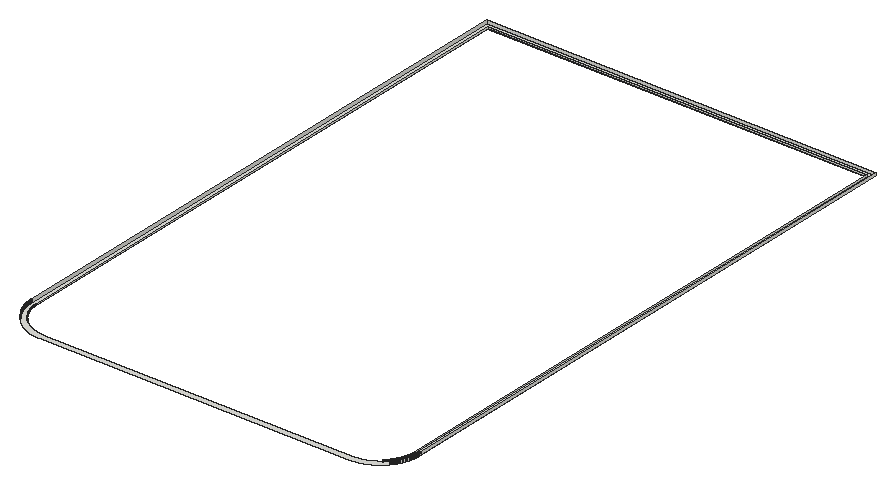
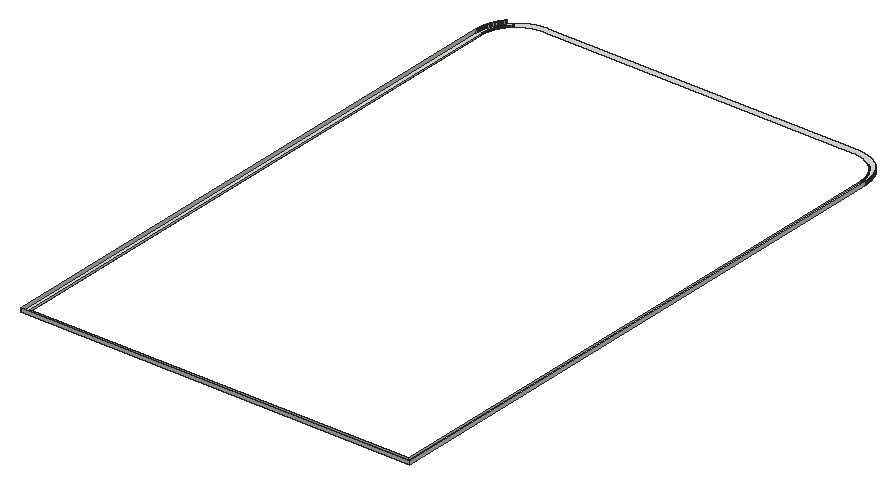
# SketchUp Ruby script. Lengths in inches.
U = 1.inch
M = Sketchup.active_model
def pt(a) = Geom::Point3d.new(a.map { |v| v * U })
def face(e, loops, mat)
  f = e.add_face(loops[0].map { |a| pt(a) })
  loops[1..].each { |l| e.add_face(l.map { |a| pt(a) }).erase! }
  f.material = f.back_material = mat if mat
  f
end
# faces: each face lists its corners as indices into pts; further lists are holes
def faces(e, pts, list, mat = nil) = list.each { |f| face(e, (f[0].is_a?(Array) ? f : [f]).map { |l| l.map { |i| pts[i] } }, mat) }
# xy, xz, yz: faces in a plane at the given z, y or x. An outline is a flat list of corners, or four numbers for a rectangle; further outlines are holes
def ring(l) = l.size == 4 ? [[l[0], l[1]], [l[2], l[1]], [l[2], l[3]], [l[0], l[3]]] : l.each_slice(2).to_a
def flat(e, list, mat, &to3) = list.each { |f| face(e, (f[0].is_a?(Array) ? f : [f]).map { |l| ring(l).map { |u, v| to3.(u, v) } }, mat) }
def xy(e, z, list, mat = nil) = flat(e, list, mat) { |x, y| [x, y, z] }
def xz(e, y, list, mat = nil) = flat(e, list, mat) { |x, z| [x, y, z] }
def yz(e, x, list, mat = nil) = flat(e, list, mat) { |y, z| [x, y, z] }
def lines(e, pts, list) = list.each { |a, b| e.add_line(pt(pts[a]), pt(pts[b])) }
# prism: a flat outline (further loops are holes) pulled along v
def prism(e, loops, v, mat = nil)
  f = face(e, loops, mat); d = Geom::Vector3d.new(v.map { |x| x * U })
  f.pushpull(f.normal.samedirection?(d) ? d.length : -d.length)
end
def box(e, o, s, mat = nil) = prism(e, [[o, [o[0] + s[0], o[1], o[2]], [o[0] + s[0], o[1] + s[1], o[2]], [o[0], o[1] + s[1], o[2]]]], [0, 0, s[2]], mat)
def at(x, y, z, deg = 0) = Geom::Transformation.translation(pt([x, y, z])) * Geom::Transformation.rotation(ORIGIN, Z_AXIS, deg.degrees)
def axes(o, x, y, z) = Geom::Transformation.new([*x, 0, *y, 0, *z, 0, *pt(o).to_a, 1])
def part(name) = M.definitions.add(name)
# library, detail: a bought-in or finely detailed component or shape, given as its bounding box
def library(name, o, s) = part(name).tap { |d| box(d.entities, o, s) }
def detail(e, o, s) = box(e.add_group.entities, o, s)
def put(e, d, t, mat = nil) = e.add_instance(d, t).tap { |i| i.material = mat if mat }
def group(e, t, mat = nil) = e.add_group.tap { |g| g.transformation = t; g.material = mat if mat }.entities
root = M.entities
xy(root,347,[[[38.61,204,38.21,204.01,37.82,204.02,37.43,204.04,37.04,204.0625,36.65,204.09,36.25,204.125,35.86,204.16,35.08,204.26,34.7,204.31,33.92,204.43,33.53,204.5,33.15,204.58,32.76,204.66,32.38,204.74,31.62,204.92,31.24,205.02,30.86,205.125,30.48,205.24,30.1,205.35,29.36,205.59,28.62,205.85,28.25,205.99,27.88,206.14,27.52,206.28,27.16,206.4375,26.8,206.59,26.44,206.76,26.08,206.92,25.73,207.09,25.03,207.45,24.69,207.64,24.34,207.83,24,208.02,23.66,208.22,23.33,208.42,22.99,208.63,22.66,208.84,22.33,209.06,22.01,209.28,21.6875,209.5,21.37,209.73,21.05,209.96,20.43,210.44,20.12,210.6875,19.82,210.93,19.52,211.1875,19.22,211.44,18.93,211.71,18.64,211.97,18.35,212.24,18.07,212.51,17.51,213.07,17.24,213.35,16.97,213.64,16.71,213.93,16.44,214.22,16.1875,214.52,15.93,214.82,15.6875,215.12,15.44,215.43,14.96,216.05,14.73,216.37,14.5,216.6875,14.28,217.01,14.06,217.33,13.84,217.66,13.63,217.99,13.42,218.33,13.22,218.66,13.02,219,12.83,219.34,12.64,219.69,12.45,220.03,12.09,220.73,11.92,221.08,11.76,221.44,11.59,221.8,11.4375,222.16,11.28,222.52,11.14,222.88,10.99,223.25,10.85,223.62,10.59,224.36,10.35,225.1,10.24,225.48,10.125,225.86,10.02,226.24,9.92,226.62,9.74,227.38,9.66,227.76,9.58,228.15,9.5,228.53,9.43,228.92,9.31,229.7,9.26,230.08,9.16,230.86,9.125,231.25,9.09,231.65,9.0625,232.04,9.04,232.43,9.02,232.82,9.01,233.21,9,233.61,9,660,300,660,300,233.61,299.99,233.21,299.98,232.82,299.96,232.43,299.9375,232.04,299.91,231.65,299.875,231.25,299.84,230.86,299.74,230.08,299.69,229.7,299.57,228.92,299.5,228.53,299.42,228.15,299.34,227.76,299.26,227.38,299.08,226.62,298.98,226.24,298.875,225.86,298.76,225.48,298.65,225.1,298.41,224.36,298.15,223.62,298.01,223.25,297.86,222.88,297.72,222.52,297.5625,222.16,297.41,221.8,297.24,221.44,297.08,221.08,296.91,220.73,296.55,220.03,296.36,219.69,296.17,219.34,295.98,219,295.78,218.66,295.58,218.33,295.37,217.99,295.16,217.66,294.94,217.33,294.72,217.01,294.5,216.6875,294.27,216.37,294.04,216.05,293.56,215.43,293.3125,215.12,293.07,214.82,292.8125,214.52,292.56,214.22,292.29,213.93,292.03,213.64,291.76,213.35,291.49,213.07,290.93,212.51,290.65,212.24,290.36,211.97,290.07,211.71,289.78,211.44,289.48,211.1875,289.18,210.93,288.88,210.6875,288.57,210.44,287.95,209.96,287.63,209.73,287.3125,209.5,286.99,209.28,286.67,209.06,286.34,208.84,286.01,208.63,285.67,208.42,285.34,208.22,285,208.02,284.66,207.83,284.31,207.64,283.97,207.45,283.27,207.09,282.92,206.92,282.56,206.76,282.2,206.59,281.84,206.4375,281.48,206.28,281.12,206.14,280.75,205.99,280.38,205.85,279.64,205.59,278.9,205.35,278.52,205.24,278.14,205.125,277.76,205.02,277.38,204.92,276.62,204.74,276.24,204.66,275.85,204.58,275.47,204.5,275.08,204.43,274.3,204.31,273.92,204.26,273.14,204.16,272.75,204.125,272.35,204.09,271.96,204.0625,271.57,204.04,271.18,204.02,270.79,204.01,270.39,204],[38.66,208,270.34,208,271.02,208.02,272.04,208.08,272.72,208.14,273.06,208.18,273.39,208.22,274.07,208.32,274.4,208.375,274.74,208.44,275.07,208.5,275.41,208.57,275.74,208.64,276.4,208.8,277.06,208.98,277.38,209.07,277.71,209.17,278.03,209.27,278.36,209.38,278.68,209.49,279.32,209.73,279.63,209.85,279.95,209.98,280.26,210.11,280.58,210.25,280.89,210.39,281.19,210.53,281.5,210.68,281.8,210.83,282.11,210.99,282.41,211.15,282.7,211.32,283,211.48,283.29,211.66,283.58,211.83,283.875,212.01,284.16,212.19,284.44,212.38,284.73,212.57,285.01,212.77,285.28,212.97,285.56,213.17,285.83,213.37,286.1,213.58,286.36,213.79,286.89,214.23,287.14,214.45,287.4,214.68,287.9,215.14,288.14,215.375,288.38,215.62,288.625,215.86,288.86,216.1,289.32,216.6,289.55,216.86,289.77,217.11,290.21,217.64,290.42,217.9,290.63,218.17,290.83,218.44,291.03,218.72,291.23,218.99,291.43,219.27,291.62,219.56,291.81,219.84,291.99,220.125,292.17,220.42,292.34,220.71,292.52,221,292.68,221.3,292.85,221.59,293.01,221.89,293.17,222.2,293.32,222.5,293.47,222.81,293.61,223.11,293.75,223.42,293.89,223.74,294.02,224.05,294.15,224.37,294.27,224.68,294.51,225.32,294.62,225.64,294.73,225.97,294.83,226.29,294.93,226.62,295.02,226.94,295.2,227.6,295.36,228.26,295.43,228.59,295.5,228.93,295.56,229.26,295.625,229.6,295.68,229.93,295.78,230.61,295.82,230.94,295.86,231.28,295.92,231.96,295.98,232.98,296,233.66,296,656,13,656,13,233.66,13.02,232.98,13.08,231.96,13.14,231.28,13.18,230.94,13.22,230.61,13.32,229.93,13.375,229.6,13.44,229.26,13.5,228.93,13.57,228.59,13.64,228.26,13.8,227.6,13.98,226.94,14.07,226.62,14.17,226.29,14.27,225.97,14.38,225.64,14.49,225.32,14.73,224.68,14.85,224.37,14.98,224.05,15.11,223.74,15.25,223.42,15.39,223.11,15.53,222.81,15.68,222.5,15.83,222.2,15.99,221.89,16.15,221.59,16.32,221.3,16.48,221,16.66,220.71,16.83,220.42,17.01,220.125,17.19,219.84,17.38,219.56,17.57,219.27,17.77,218.99,17.97,218.72,18.17,218.44,18.37,218.17,18.58,217.9,18.79,217.64,19.23,217.11,19.45,216.86,19.68,216.6,20.14,216.1,20.375,215.86,20.62,215.62,20.86,215.375,21.1,215.14,21.6,214.68,21.86,214.45,22.11,214.23,22.64,213.79,22.9,213.58,23.17,213.37,23.44,213.17,23.72,212.97,23.99,212.77,24.27,212.57,24.56,212.38,24.84,212.19,25.125,212.01,25.42,211.83,25.71,211.66,26,211.48,26.3,211.32,26.59,211.15,26.89,210.99,27.2,210.83,27.5,210.68,27.81,210.53,28.11,210.39,28.42,210.25,28.74,210.11,29.05,209.98,29.37,209.85,29.68,209.73,30.32,209.49,30.64,209.38,30.97,209.27,31.29,209.17,31.62,209.07,31.94,208.98,32.6,208.8,33.26,208.64,33.59,208.57,33.93,208.5,34.26,208.44,34.6,208.375,34.93,208.32,35.61,208.22,35.94,208.18,36.28,208.14,36.96,208.08,37.98,208.02]]])
xz(root,656,[[13,347,296,348]])
xz(root,660,[[9,347,300,349.5]])
yz(root,9,[[233.61,347,234,349.5],[234,347,660,349.5]])
yz(root,13,[[233.66,347,234,348],[234,347,656,348]])
yz(root,296,[[233.66,347,234,348],[234,347,656,348]])
yz(root,300,[[233.61,347,234,349.5],[234,347,660,349.5]])
p = [[16.1875,214.52,349.5],[15.93,214.82,349.5],[15.93,214.82,347],[16.1875,214.52,347],[21.86,214.45,347],[21.6,214.68,347],
  [21.6,214.68,348],[21.86,214.45,348],[287.4,214.68,347],[287.14,214.45,347],[287.14,214.45,348],[287.4,214.68,348],
  [293.07,214.82,349.5],[292.8125,214.52,349.5],[292.8125,214.52,347],[293.07,214.82,347],[21.35,214.91,347],[21.35,214.91,348],
  [287.65,214.91,347],[287.65,214.91,348],[15.6875,215.12,349.5],[15.6875,215.12,347],[293.3125,215.12,349.5],[293.3125,215.12,347],
  [21.1,215.14,347],[21.1,215.14,348],[287.9,215.14,347],[287.9,215.14,348],[15.44,215.43,349.5],[15.44,215.43,347],
  [20.86,215.375,347],[20.86,215.375,348],[288.14,215.375,347],[288.14,215.375,348],[293.56,215.43,349.5],[293.56,215.43,347],
  [15.2,215.74,349.5],[15.2,215.74,347],[20.62,215.62,347],[20.62,215.62,348],[288.38,215.62,347],[288.38,215.62,348],
  [293.8,215.74,349.5],[293.8,215.74,347],[20.375,215.86,347],[20.375,215.86,348],[288.625,215.86,347],[288.625,215.86,348],
  [14.96,216.05,349.5],[14.96,216.05,347],[294.04,216.05,349.5],[294.04,216.05,347],[20.14,216.1,347],[20.14,216.1,348],
  [288.86,216.1,347],[288.86,216.1,348],[14.73,216.37,349.5],[14.73,216.37,347],[19.91,216.35,347],[19.91,216.35,348],
  [289.09,216.35,347],[289.09,216.35,348],[294.27,216.37,349.5],[294.27,216.37,347],[14.5,216.6875,349.5],[14.5,216.6875,347],
  [19.68,216.6,347],[19.68,216.6,348],[289.32,216.6,347],[289.32,216.6,348],[294.5,216.6875,349.5],[294.5,216.6875,347],
  [19.45,216.86,347],[19.45,216.86,348],[289.55,216.86,347],[289.55,216.86,348],[14.28,217.01,349.5],[14.28,217.01,347],
  [294.72,217.01,349.5],[294.72,217.01,347],[19.23,217.11,347],[19.23,217.11,348],[289.77,217.11,347],[289.77,217.11,348],
  [14.06,217.33,349.5],[14.06,217.33,347],[294.94,217.33,349.5],[294.94,217.33,347],[19.01,217.375,347],[19.01,217.375,348],
  [289.99,217.375,347],[289.99,217.375,348],[13.84,217.66,349.5],[13.84,217.66,347],[295.16,217.66,349.5],[295.16,217.66,347],
  [18.79,217.64,347],[18.79,217.64,348],[290.21,217.64,347],[290.21,217.64,348],[18.58,217.9,347],[18.58,217.9,348],
  [290.42,217.9,347],[290.42,217.9,348],[13.63,217.99,349.5],[13.63,217.99,347],[295.37,217.99,349.5],[295.37,217.99,347],
  [18.37,218.17,347],[18.37,218.17,348],[290.63,218.17,347],[290.63,218.17,348],[13.42,218.33,349.5],[13.42,218.33,347],
  [295.58,218.33,349.5],[295.58,218.33,347],[18.17,218.44,347],[18.17,218.44,348],[290.83,218.44,347],[290.83,218.44,348],
  [13.22,218.66,349.5],[13.22,218.66,347],[295.78,218.66,349.5],[295.78,218.66,347],[17.97,218.72,347],[17.97,218.72,348],
  [291.03,218.72,347],[291.03,218.72,348],[13.02,219,349.5],[13.02,219,347],[17.77,218.99,347],[17.77,218.99,348],
  [291.23,218.99,347],[291.23,218.99,348],[295.98,219,349.5],[295.98,219,347],[12.83,219.34,349.5],[12.83,219.34,347],
  [17.57,219.27,347],[17.57,219.27,348],[291.43,219.27,347],[291.43,219.27,348],[296.17,219.34,349.5],[296.17,219.34,347],
  [12.64,219.69,349.5],[12.64,219.69,347],[17.38,219.56,347],[17.38,219.56,348],[291.62,219.56,347],[291.62,219.56,348],
  [296.36,219.69,349.5],[296.36,219.69,347],[17.19,219.84,347],[17.19,219.84,348],[291.81,219.84,347],[291.81,219.84,348],
  [12.45,220.03,349.5],[12.45,220.03,347],[296.55,220.03,349.5],[296.55,220.03,347],[17.01,220.125,347],[17.01,220.125,348],
  [291.99,220.125,347],[291.99,220.125,348],[12.27,220.38,349.5],[12.27,220.38,347],[296.73,220.38,349.5],[296.73,220.38,347],
  [16.83,220.42,347],[16.83,220.42,348],[292.17,220.42,347],[292.17,220.42,348],[12.09,220.73,349.5],[12.09,220.73,347],
  [16.66,220.71,347],[16.66,220.71,348],[292.34,220.71,347],[292.34,220.71,348],[296.91,220.73,349.5],[296.91,220.73,347],
  [11.92,221.08,349.5],[11.92,221.08,347],[16.48,221,347],[16.48,221,348],[292.52,221,347],[292.52,221,348],
  [297.08,221.08,349.5],[297.08,221.08,347],[16.32,221.3,347],[16.32,221.3,348],[292.68,221.3,347],[292.68,221.3,348],
  [11.76,221.44,349.5],[11.76,221.44,347],[297.24,221.44,349.5],[297.24,221.44,347],[16.15,221.59,347],[16.15,221.59,348],
  [292.85,221.59,347],[292.85,221.59,348],[11.59,221.8,349.5],[11.59,221.8,347],[297.41,221.8,349.5],[297.41,221.8,347],
  [15.99,221.89,347],[15.99,221.89,348],[293.01,221.89,347],[293.01,221.89,348],[11.4375,222.16,349.5],[11.4375,222.16,347],
  [297.5625,222.16,349.5],[297.5625,222.16,347],[15.83,222.2,347],[15.83,222.2,348],[293.17,222.2,347],[293.17,222.2,348],
  [11.28,222.52,349.5],[11.28,222.52,347],[15.68,222.5,347],[15.68,222.5,348],[293.32,222.5,347],[293.32,222.5,348],
  [297.72,222.52,349.5],[297.72,222.52,347],[11.14,222.88,349.5],[11.14,222.88,347],[15.53,222.81,347],[15.53,222.81,348],
  [293.47,222.81,347],[293.47,222.81,348],[297.86,222.88,349.5],[297.86,222.88,347],[15.39,223.11,347],[15.39,223.11,348],
  [293.61,223.11,347],[293.61,223.11,348],[10.99,223.25,349.5],[10.99,223.25,347],[298.01,223.25,349.5],[298.01,223.25,347],
  [15.25,223.42,347],[15.25,223.42,348],[293.75,223.42,347],[293.75,223.42,348],[10.85,223.62,349.5],[10.85,223.62,347],
  [298.15,223.62,349.5],[298.15,223.62,347],[15.11,223.74,347],[15.11,223.74,348],[293.89,223.74,347],[293.89,223.74,348],
  [10.72,223.99,349.5],[10.72,223.99,347],[298.28,223.99,349.5],[298.28,223.99,347],[14.98,224.05,347],[14.98,224.05,348],
  [294.02,224.05,347],[294.02,224.05,348],[10.59,224.36,349.5],[10.59,224.36,347],[298.41,224.36,349.5],[298.41,224.36,347],
  [14.85,224.37,347],[14.85,224.37,348],[294.15,224.37,347],[294.15,224.37,348],[10.47,224.73,349.5],[10.47,224.73,347],
  [14.73,224.68,347],[14.73,224.68,348],[294.27,224.68,347],[294.27,224.68,348],[298.53,224.73,349.5],[298.53,224.73,347],
  [10.35,225.1,349.5],[10.35,225.1,347],[14.61,225,347],[14.61,225,348],[294.39,225,347],[294.39,225,348],
  [298.65,225.1,349.5],[298.65,225.1,347],[14.49,225.32,347],[14.49,225.32,348],[294.51,225.32,347],[294.51,225.32,348],
  [10.24,225.48,349.5],[10.24,225.48,347],[298.76,225.48,349.5],[298.76,225.48,347],[14.38,225.64,347],[14.38,225.64,348],
  [294.62,225.64,347],[294.62,225.64,348],[10.125,225.86,349.5],[10.125,225.86,347],[298.875,225.86,349.5],[298.875,225.86,347],
  [14.27,225.97,347],[14.27,225.97,348],[294.73,225.97,347],[294.73,225.97,348],[10.02,226.24,349.5],[10.02,226.24,347],
  [298.98,226.24,349.5],[298.98,226.24,347],[14.17,226.29,347],[14.17,226.29,348],[294.83,226.29,347],[294.83,226.29,348],
  [9.92,226.62,349.5],[9.92,226.62,347],[299.08,226.62,349.5],[299.08,226.62,347],[14.07,226.62,347],[14.07,226.62,348],
  [294.93,226.62,347],[294.93,226.62,348],[9.83,227,349.5],[9.83,227,347],[13.98,226.94,347],[13.98,226.94,348],
  [295.02,226.94,347],[295.02,226.94,348],[299.17,227,349.5],[299.17,227,347],[13.89,227.27,347],[13.89,227.27,348],
  [295.11,227.27,347],[295.11,227.27,348],[9.74,227.38,349.5],[9.74,227.38,347],[299.26,227.38,349.5],[299.26,227.38,347],
  [13.8,227.6,347],[13.8,227.6,348],[295.2,227.6,347],[295.2,227.6,348],[9.66,227.76,349.5],[9.66,227.76,347],
  [299.34,227.76,349.5],[299.34,227.76,347],[13.72,227.93,347],[13.72,227.93,348],[295.28,227.93,347],[295.28,227.93,348],
  [9.58,228.15,349.5],[9.58,228.15,347],[299.42,228.15,349.5],[299.42,228.15,347],[13.64,228.26,347],[13.64,228.26,348],
  [295.36,228.26,347],[295.36,228.26,348],[9.5,228.53,349.5],[9.5,228.53,347],[299.5,228.53,349.5],[299.5,228.53,347],
  [13.57,228.59,347],[13.57,228.59,348],[295.43,228.59,347],[295.43,228.59,348],[9.43,228.92,349.5],[9.43,228.92,347],
  [299.57,228.92,349.5],[299.57,228.92,347],[13.5,228.93,347],[13.5,228.93,348],[295.5,228.93,347],[295.5,228.93,348],
  [9.37,229.31,349.5],[9.37,229.31,347],[13.44,229.26,347],[13.44,229.26,348],[295.56,229.26,347],[295.56,229.26,348],
  [299.63,229.31,349.5],[299.63,229.31,347],[9.31,229.7,349.5],[9.31,229.7,347],[13.375,229.6,347],[13.375,229.6,348],
  [295.625,229.6,347],[295.625,229.6,348],[299.69,229.7,349.5],[299.69,229.7,347],[13.32,229.93,347],[13.32,229.93,348],
  [295.68,229.93,347],[295.68,229.93,348],[9.26,230.08,349.5],[9.26,230.08,347],[299.74,230.08,349.5],[299.74,230.08,347],
  [13.27,230.27,347],[13.27,230.27,348],[295.73,230.27,347],[295.73,230.27,348],[9.21,230.47,349.5],[9.21,230.47,347],
  [299.79,230.47,349.5],[299.79,230.47,347],[13.22,230.61,347],[13.22,230.61,348],[295.78,230.61,347],[295.78,230.61,348],
  [9.16,230.86,349.5],[9.16,230.86,347],[299.84,230.86,349.5],[299.84,230.86,347],[13.18,230.94,347],[13.18,230.94,348],
  [295.82,230.94,347],[295.82,230.94,348],[9.125,231.25,349.5],[9.125,231.25,347],[13.14,231.28,347],[13.14,231.28,348],
  [295.86,231.28,347],[295.86,231.28,348],[299.875,231.25,349.5],[299.875,231.25,347],[9.09,231.65,349.5],[9.09,231.65,347],
  [13.11,231.62,347],[13.11,231.62,348],[295.89,231.62,347],[295.89,231.62,348],[299.91,231.65,349.5],[299.91,231.65,347],
  [9.0625,232.04,349.5],[9.0625,232.04,347],[13.08,231.96,347],[13.08,231.96,348],[295.92,231.96,347],[295.92,231.96,348],
  [299.9375,232.04,349.5],[299.9375,232.04,347],[9.04,232.43,349.5],[9.04,232.43,347],[13.06,232.3,347],[13.06,232.3,348],
  [295.94,232.3,347],[295.94,232.3,348],[299.96,232.43,349.5],[299.96,232.43,347],[13.04,232.64,347],[13.04,232.64,348],
  [295.96,232.64,347],[295.96,232.64,348],[9.02,232.82,349.5],[9.02,232.82,347],[299.98,232.82,349.5],[299.98,232.82,347],
  [13.02,232.98,347],[13.02,232.98,348],[295.98,232.98,347],[295.98,232.98,348],[9.01,233.21,349.5],[9.01,233.21,347],
  [299.99,233.21,349.5],[299.99,233.21,347],[13.01,233.32,347],[13.01,233.32,348],[295.99,233.32,347],[295.99,233.32,348],
  [9,233.61,349.5],[9,233.61,347],[300,233.61,349.5],[300,233.61,347],[13,233.66,347],[13,233.66,348],
  [296,233.66,347],[296,233.66,348]]
faces(root,p,[[0,1,2,3],[4,5,6,7],[8,9,10,11],[12,13,14,15],[5,16,17,6],[18,8,11,19],[1,20,21,2],[22,12,15,23],
  [16,24,25,17],[26,18,19,27],[20,28,29,21],[24,30,31,25],[32,26,27,33],[34,22,23,35],[28,36,37,29],[30,38,39,31],
  [40,32,33,41],[42,34,35,43],[38,44,45,39],[46,40,41,47],[36,48,49,37],[50,42,43,51],[44,52,53,45],[54,46,47,55],
  [48,56,57,49],[52,58,59,53],[60,54,55,61],[62,50,51,63],[56,64,65,57],[58,66,67,59],[68,60,61,69],[70,62,63,71],
  [66,72,73,67],[74,68,69,75],[64,76,77,65],[78,70,71,79],[72,80,81,73],[82,74,75,83],[76,84,85,77],[86,78,79,87],
  [80,88,89,81],[90,82,83,91],[84,92,93,85],[94,86,87,95],[88,96,97,89],[98,90,91,99],[96,100,101,97],[102,98,99,103],
  [92,104,105,93],[106,94,95,107],[100,108,109,101],[110,102,103,111],[104,112,113,105],[114,106,107,115],[108,116,117,109],[118,110,111,119],
  [112,120,121,113],[122,114,115,123],[116,124,125,117],[126,118,119,127],[120,128,129,121],[124,130,131,125],[132,126,127,133],[134,122,123,135],
  [128,136,137,129],[130,138,139,131],[140,132,133,141],[142,134,135,143],[136,144,145,137],[138,146,147,139],[148,140,141,149],[150,142,143,151],
  [146,152,153,147],[154,148,149,155],[144,156,157,145],[158,150,151,159],[152,160,161,153],[162,154,155,163],[156,164,165,157],[166,158,159,167],
  [160,168,169,161],[170,162,163,171],[164,172,173,165],[168,174,175,169],[176,170,171,177],[178,166,167,179],[172,180,181,173],[174,182,183,175],
  [184,176,177,185],[186,178,179,187],[182,188,189,183],[190,184,185,191],[180,192,193,181],[194,186,187,195],[188,196,197,189],[198,190,191,199],
  [192,200,201,193],[202,194,195,203],[196,204,205,197],[206,198,199,207],[200,208,209,201],[210,202,203,211],[204,212,213,205],[214,206,207,215],
  [208,216,217,209],[212,218,219,213],[220,214,215,221],[222,210,211,223],[216,224,225,217],[218,226,227,219],[228,220,221,229],[230,222,223,231],
  [226,232,233,227],[234,228,229,235],[224,236,237,225],[238,230,231,239],[232,240,241,233],[242,234,235,243],[236,244,245,237],[246,238,239,247],
  [240,248,249,241],[250,242,243,251],[244,252,253,245],[254,246,247,255],[248,256,257,249],[258,250,251,259],[252,260,261,253],[262,254,255,263],
  [256,264,265,257],[266,258,259,267],[260,268,269,261],[264,270,271,265],[272,266,267,273],[274,262,263,275],[268,276,277,269],[270,278,279,271],
  [280,272,273,281],[282,274,275,283],[278,284,285,279],[286,280,281,287],[276,288,289,277],[290,282,283,291],[284,292,293,285],[294,286,287,295],
  [288,296,297,289],[298,290,291,299],[292,300,301,293],[302,294,295,303],[296,304,305,297],[306,298,299,307],[300,308,309,301],[310,302,303,311],
  [304,312,313,305],[314,306,307,315],[308,316,317,309],[318,310,311,319],[312,320,321,313],[316,322,323,317],[324,318,319,325],[326,314,315,327],
  [322,328,329,323],[330,324,325,331],[320,332,333,321],[334,326,327,335],[328,336,337,329],[338,330,331,339],[332,340,341,333],[342,334,335,343],
  [336,344,345,337],[346,338,339,347],[340,348,349,341],[350,342,343,351],[344,352,353,345],[354,346,347,355],[348,356,357,349],[358,350,351,359],
  [352,360,361,353],[362,354,355,363],[356,364,365,357],[366,358,359,367],[360,368,369,361],[370,362,363,371],[364,372,373,365],[368,374,375,369],
  [376,370,371,377],[378,366,367,379],[372,380,381,373],[374,382,383,375],[384,376,377,385],[386,378,379,387],[382,388,389,383],[390,384,385,391],
  [380,392,393,381],[394,386,387,395],[388,396,397,389],[398,390,391,399],[392,400,401,393],[402,394,395,403],[396,404,405,397],[406,398,399,407],
  [400,408,409,401],[410,402,403,411],[404,412,413,405],[414,406,407,415],[408,416,417,409],[412,418,419,413],[420,414,415,421],[422,410,411,423],
  [416,424,425,417],[418,426,427,419],[428,420,421,429],[430,422,423,431],[424,432,433,425],[426,434,435,427],[436,428,429,437],[438,430,431,439],
  [432,440,441,433],[434,442,443,435],[444,436,437,445],[446,438,439,447],[442,448,449,443],[450,444,445,451],[440,452,453,441],[454,446,447,455],
  [448,456,457,449],[458,450,451,459],[452,460,461,453],[462,454,455,463],[456,464,465,457],[466,458,459,467],[460,468,469,461],[470,462,463,471],
  [464,472,473,465],[474,466,467,475]])
